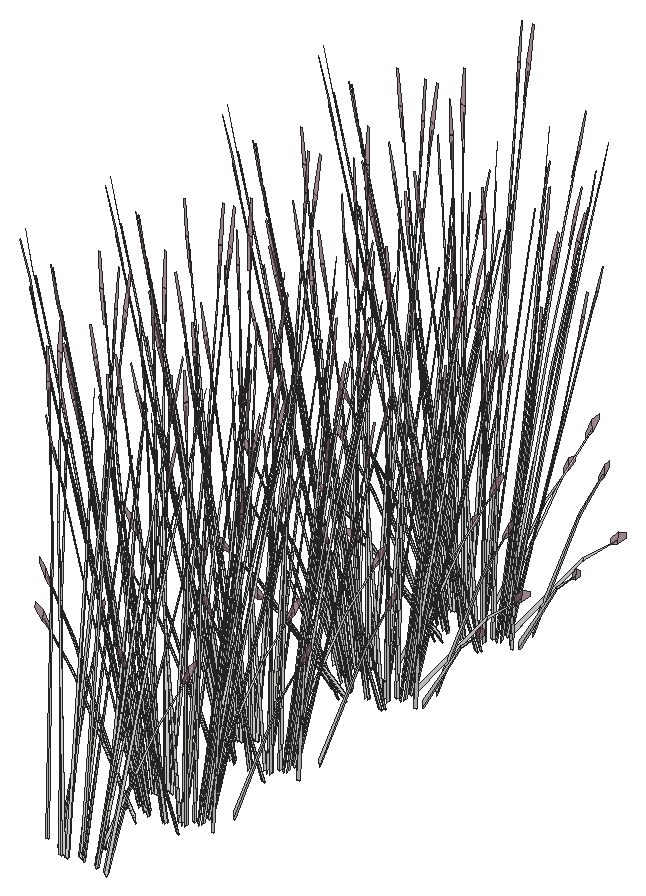
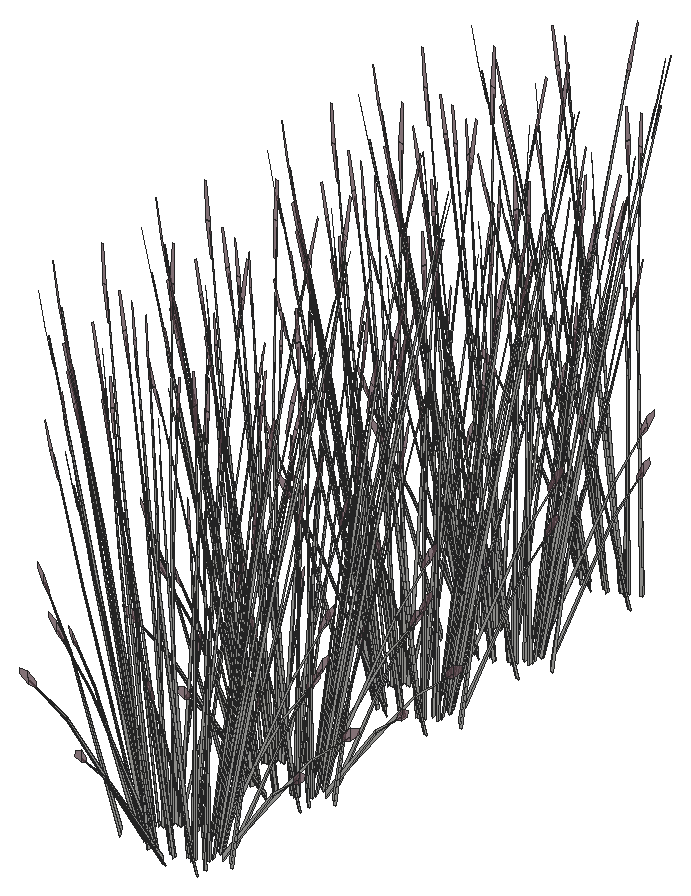
# SketchUp Ruby script. Lengths in inches.
U = 1.inch
M = Sketchup.active_model
def pt(a) = Geom::Point3d.new(a.map { |v| v * U })
def face(e, loops, mat)
  f = e.add_face(loops[0].map { |a| pt(a) })
  loops[1..].each { |l| e.add_face(l.map { |a| pt(a) }).erase! }
  f.material = f.back_material = mat if mat
  f
end
# faces: each face lists its corners as indices into pts; further lists are holes
def faces(e, pts, list, mat = nil) = list.each { |f| face(e, (f[0].is_a?(Array) ? f : [f]).map { |l| l.map { |i| pts[i] } }, mat) }
# xy, xz, yz: faces in a plane at the given z, y or x. An outline is a flat list of corners, or four numbers for a rectangle; further outlines are holes
def ring(l) = l.size == 4 ? [[l[0], l[1]], [l[2], l[1]], [l[2], l[3]], [l[0], l[3]]] : l.each_slice(2).to_a
def flat(e, list, mat, &to3) = list.each { |f| face(e, (f[0].is_a?(Array) ? f : [f]).map { |l| ring(l).map { |u, v| to3.(u, v) } }, mat) }
def xy(e, z, list, mat = nil) = flat(e, list, mat) { |x, y| [x, y, z] }
def xz(e, y, list, mat = nil) = flat(e, list, mat) { |x, z| [x, y, z] }
def yz(e, x, list, mat = nil) = flat(e, list, mat) { |y, z| [x, y, z] }
def lines(e, pts, list) = list.each { |a, b| e.add_line(pt(pts[a]), pt(pts[b])) }
# prism: a flat outline (further loops are holes) pulled along v
def prism(e, loops, v, mat = nil)
  f = face(e, loops, mat); d = Geom::Vector3d.new(v.map { |x| x * U })
  f.pushpull(f.normal.samedirection?(d) ? d.length : -d.length)
end
def box(e, o, s, mat = nil) = prism(e, [[o, [o[0] + s[0], o[1], o[2]], [o[0] + s[0], o[1] + s[1], o[2]], [o[0], o[1] + s[1], o[2]]]], [0, 0, s[2]], mat)
def at(x, y, z, deg = 0) = Geom::Transformation.translation(pt([x, y, z])) * Geom::Transformation.rotation(ORIGIN, Z_AXIS, deg.degrees)
def axes(o, x, y, z) = Geom::Transformation.new([*x, 0, *y, 0, *z, 0, *pt(o).to_a, 1])
def part(name) = M.definitions.add(name)
# library, detail: a bought-in or finely detailed component or shape, given as its bounding box
def library(name, o, s) = part(name).tap { |d| box(d.entities, o, s) }
def detail(e, o, s) = box(e.add_group.entities, o, s)
def put(e, d, t, mat = nil) = e.add_instance(d, t).tap { |i| i.material = mat if mat }
def group(e, t, mat = nil) = e.add_group.tap { |g| g.transformation = t; g.material = mat if mat }.entities
root = M.entities
M.materials.add("LightPink_Translucent").color = [144, 107, 117]
M.materials["LightPink_Translucent"].alpha = 0.75
c1 = part("blade")
p = [[2.15,0.21,22],[0,0.17,0],[0.09,0.45,0],[2.18,0.31,22],[2.29,0.31,22],[0.38,0.45,0],
  [2.48,0.24,33],[2.49,0.24,33],[2.48,0.22,33]]
faces(c1.entities,p,[[0,1,2,3],[4,5,2,3],[6,3,4,7],[8,0,3,6]])
c2 = part("seeds")
p = [[0.3,-0.1,1.38],[-0.01,-0.03,1.59],[-0.01,-0.03,0.03],[0.14,-0.07,-0.07],[0.29,-0.03,3],[0.15,0.01,3.11]]
faces(c2.entities,p,[[0,1,2,3],[1,0,4,5]],"LightPink_Translucent")
c3 = part("blade with seeds")
put(c3.entities,c1,at(0,0,0))
put(c3.entities,c2,axes([2.4,0.25,30.99],[1.5799,-0.05474,1.17369],[-0.12525,1.92788,0.29478],[-0.07173,-0.02425,1.56792]))
put(root,c3,axes([335.62,462.02,52.18],[-0.02542,0.29714,0.05682],[-0.38391,-0.00815,0.44729],[0.14706,0.03109,0.68204]))
put(root,c3,axes([335.65,461.93,52.18],[-0.3723,0.25748,0.42415],[-0.32109,-0.27343,0.34973],[0.17467,0.04749,0.87768]))
put(root,c3,axes([330.85,462.21,52.99],[0.44556,0.1043,-0.05733],[-0.13706,0.32103,-0.25992],[-0.07288,0.04874,0.85731]))
put(root,c3,axes([334.47,462.22,52.46],[-0.07798,-0.31474,0.31292],[0.44579,-0.08311,-0.40398],[0.11974,0.09019,0.77298]))
put(root,c3,axes([332.45,461.94,52.46],[0.34164,-0.20573,0.31292],[0.3234,0.23491,-0.40398],[-0.04921,0.11936,0.77298]))
put(root,c3,axes([334.04,462.66,52.16],[0.00149,-0.04731,1.56736],[0.4327,-0.20872,-0.1481],[0.1503,0.0745,0.27737]))
put(root,c3,axes([332.14,462.12,52.18],[-0.41493,-0.01821,0.05682],[0.01138,-0.27493,0.44729],[-0.04342,0.10531,0.68204]))
put(root,c3,axes([332.27,462.15,52.18],[-0.35954,-0.26661,0.42415],[0.38183,-0.22994,0.34973],[-0.06632,0.12508,0.87768]))
put(root,c3,axes([333.4,462.27,52.46],[0.15222,-0.30049,0.31292],[0.44409,0.08764,-0.40398],[0.04072,0.12098,0.77298]))
put(root,c3,axes([334.54,462.51,52.18],[-0.22948,0.24822,0.05682],[-0.32679,-0.14452,0.44729],[0.10565,0.07958,0.68204]))
put(root,c3,axes([334,463.35,52.99],[0.34892,-0.22417,-0.05733],[0.3197,0.24551,-0.25992],[0.02251,0.06957,0.85731]))
put(root,c3,axes([334.64,462.44,52.18],[-0.5022,0.08967,0.42415],[-0.08716,-0.35177,0.34973],[0.11811,0.10367,0.87768]))
put(root,c3,axes([333.27,462.55,52.18],[-0.37205,0.1328,0.05682],[-0.18211,-0.24217,0.44729],[0.03593,0.10675,0.68204]))
put(root,c3,axes([332.23,461.99,52.77],[0.55492,0.01936,-0.11927],[-0.01517,0.36657,-0.66198],[-0.03855,0.14118,1.00587]))
put(root,c3,axes([333.4,462.52,52.47],[-0.49753,-0.10215,0.47081],[0.17013,-0.33585,0.3882],[0.0299,0.13207,0.97422]))
put(root,c3,axes([331.05,462.96,52.16],[0.05728,-0.02359,1.56736],[0.47345,0.15692,-0.1481],[-0.01113,0.13066,0.27737]))
put(root,c3,axes([335.78,468.35,52.16],[-0.05128,0.02985,1.56736],[-0.5024,-0.1007,-0.1481],[-0.01819,-0.13025,0.27737]))
put(root,c3,axes([333.05,467.78,52.16],[-0.00942,0.04684,1.56736],[-0.46458,0.16998,-0.1481],[-0.13671,-0.08689,0.27737]))
put(root,c3,axes([332.94,468.61,52.5],[0.56246,-0.10044,0.47505],[0.09762,0.39398,0.3917],[-0.13228,-0.11611,0.983]))
put(root,c3,axes([334.22,468.68,52.18],[0.49753,0.10215,0.42415],[-0.17013,0.33585,0.34973],[-0.0299,-0.13207,0.87768]))
put(root,c3,axes([334.35,468.66,52.18],[0.37205,-0.1328,0.05682],[0.18211,0.24217,0.44729],[-0.03593,-0.10675,0.68204]))
put(root,c3,axes([333.07,468.7,52.18],[0.22948,-0.24822,0.05682],[0.32679,0.14452,0.44729],[-0.10565,-0.07958,0.68204]))
put(root,c3,axes([334.21,468.93,52.46],[-0.15222,0.30049,0.31292],[-0.44409,-0.08764,-0.40398],[-0.04072,-0.12098,0.77298]))
put(root,c3,axes([335.34,469.06,52.18],[0.35954,0.26661,0.42415],[-0.38183,0.22994,0.34973],[0.06632,-0.12508,0.87768]))
put(root,c3,axes([333.18,468.67,52.8],[-0.33698,0.3746,-0.12034],[-0.48801,-0.21581,-0.66795],[-0.16964,-0.10584,1.01494]))
put(root,c3,axes([335.48,469.08,52.18],[0.41493,0.01821,0.05682],[-0.01138,0.27493,0.44729],[0.04342,-0.10531,0.68204]))
put(root,c3,axes([335.17,469.27,52.46],[-0.34164,0.20573,0.31292],[-0.3234,-0.23491,-0.40398],[0.04921,-0.11936,0.77298]))
put(root,c3,axes([333.14,468.98,52.46],[0.07798,0.31474,0.31292],[-0.44579,0.08311,-0.40398],[-0.11974,-0.09019,0.77298]))
put(root,c3,axes([331.8,469.1875,52.5],[0.41698,-0.28837,0.47505],[0.35962,0.30624,0.3917],[-0.19563,-0.05319,0.983]))
put(root,c3,axes([337.14,469.84,52.16],[-0.06595,-0.00297,1.56736],[-0.27386,-0.31799,-0.1481],[0.10998,-0.10455,0.27737]))
put(root,c3,axes([331.99,469.18,52.18],[0.02542,-0.29714,0.05682],[0.38391,0.00815,0.44729],[-0.14706,-0.03109,0.68204]))
put(root,c3,axes([335.76,469.91,52.46],[-0.43951,0.05584,0.31292],[-0.11606,-0.31924,-0.40398],[0.12595,-0.08575,0.77298]))
put(root,c3,axes([336.16,469.85,52.18],[0.34663,0.16434,0.05682],[-0.20181,0.23402,0.44729],[0.11113,-0.07566,0.68204]))
put(root,c3,axes([336.0625,469.79,52.18],[0.12522,0.35963,0.42415],[-0.49122,0.06241,0.34973],[0.14477,-0.08458,0.87768]))
put(root,c3,axes([331.47,468.8,52.16],[0.03743,0.039,1.56736],[-0.18045,0.35054,-0.1481],[-0.18276,0.00254,0.27737]))
put(root,c3,axes([332.25,469.41,52.46],[0.28729,0.24465,0.31292],[-0.32804,0.23159,-0.40398],[-0.16667,-0.03524,0.77298]))
put(root,c3,axes([335.83,470.67,52.46],[-0.41962,-0.10901,0.31292],[0.12239,-0.31802,-0.40398],[0.16894,-0.02916,0.77298]))
put(root,c3,axes([331.4375,470.09,52.18],[0.14265,-0.35629,0.42415],[0.46898,0.12183,0.34973],[-0.18443,0.02141,0.87768]))
put(root,c3,axes([331.4,469.99,52.18],[-0.18545,-0.26643,0.05682],[0.33817,-0.13041,0.44729],[-0.14907,0.02573,0.68204]))
put(root,c3,axes([336.21,470.77,52.18],[0.18545,0.26643,0.05682],[-0.33817,0.13041,0.44729],[0.14907,-0.02573,0.68204]))
put(root,c3,axes([336.18,470.67,52.18],[-0.14265,0.35629,0.42415],[-0.46898,-0.12183,0.34973],[0.18443,-0.02141,0.87768]))
put(root,c3,axes([331.78,470.09,52.46],[0.41962,0.10901,0.31292],[-0.12239,0.31802,-0.40398],[-0.16894,0.02916,0.77298]))
put(root,c3,axes([337.02,471.83,52.16],[-0.04566,-0.03421,1.56736],[0.09987,-0.36669,-0.1481],[0.17984,-0.02343,0.27737]))
put(root,c3,axes([335.36,471.35,52.46],[-0.28729,-0.24465,0.31292],[0.32804,-0.23159,-0.40398],[0.16667,0.03524,0.77298]))
put(root,c3,axes([331.55,470.97,52.18],[-0.12522,-0.35963,0.42415],[0.49122,-0.06241,0.34973],[-0.14477,0.08458,0.87768]))
put(root,c3,axes([331.45,470.91,52.18],[-0.34663,-0.16434,0.05682],[0.20181,-0.23402,0.44729],[-0.11113,0.07566,0.68204]))
put(root,c3,axes([331.85,470.86,52.46],[0.43951,-0.05584,0.31292],[0.11606,0.31924,-0.40398],[-0.12595,0.08575,0.77298]))
put(root,c3,axes([330.16,470.71,52.16],[0.06444,0.01048,1.56736],[0.19934,0.34525,-0.1481],[-0.13191,0.09062,0.27737]))
put(root,c3,axes([335.62,471.58,52.18],[-0.02542,0.29714,0.05682],[-0.38391,-0.00815,0.44729],[0.14706,0.03109,0.68204]))
put(root,c3,axes([335.65,471.48,52.18],[-0.3723,0.25748,0.42415],[-0.32109,-0.27343,0.34973],[0.17467,0.04749,0.87768]))
put(root,c3,axes([330.85,471.76,52.99],[0.44556,0.1043,-0.05733],[-0.13706,0.32103,-0.25992],[-0.07288,0.04874,0.85731]))
put(root,c3,axes([334.47,471.78,52.46],[-0.07798,-0.31474,0.31292],[0.44579,-0.08311,-0.40398],[0.11974,0.09019,0.77298]))
put(root,c3,axes([332.45,471.49,52.46],[0.34164,-0.20573,0.31292],[0.3234,0.23491,-0.40398],[-0.04921,0.11936,0.77298]))
put(root,c3,axes([334.04,472.22,52.16],[0.00149,-0.04731,1.56736],[0.4327,-0.20872,-0.1481],[0.1503,0.0745,0.27737]))
put(root,c3,axes([332.14,471.68,52.18],[-0.41493,-0.01821,0.05682],[0.01138,-0.27493,0.44729],[-0.04342,0.10531,0.68204]))
put(root,c3,axes([332.27,471.7,52.18],[-0.35954,-0.26661,0.42415],[0.38183,-0.22994,0.34973],[-0.06632,0.12508,0.87768]))
put(root,c3,axes([333.4,471.83,52.46],[0.15222,-0.30049,0.31292],[0.44409,0.08764,-0.40398],[0.04072,0.12098,0.77298]))
put(root,c3,axes([335.78,476.15,52.16],[-0.05128,0.02985,1.56736],[-0.5024,-0.1007,-0.1481],[-0.01819,-0.13025,0.27737]))
put(root,c3,axes([334.54,472.06,52.18],[-0.22948,0.24822,0.05682],[-0.32679,-0.14452,0.44729],[0.10565,0.07958,0.68204]))
put(root,c3,axes([334,472.9,52.99],[0.34892,-0.22417,-0.05733],[0.3197,0.24551,-0.25992],[0.02251,0.06957,0.85731]))
put(root,c3,axes([334.64,472,52.18],[-0.5022,0.08967,0.42415],[-0.08716,-0.35177,0.34973],[0.11811,0.10367,0.87768]))
put(root,c3,axes([333.05,475.58,52.16],[-0.00942,0.04684,1.56736],[-0.46458,0.16998,-0.1481],[-0.13671,-0.08689,0.27737]))
put(root,c3,axes([333.27,472.1,52.18],[-0.37205,0.1328,0.05682],[-0.18211,-0.24217,0.44729],[0.03593,0.10675,0.68204]))
put(root,c3,axes([332.23,471.55,52.77],[0.55492,0.01936,-0.11927],[-0.01517,0.36657,-0.66198],[-0.03855,0.14118,1.00587]))
put(root,c3,axes([332.94,476.41,52.5],[0.56246,-0.10044,0.47505],[0.09762,0.39398,0.3917],[-0.13228,-0.11611,0.983]))
put(root,c3,axes([333.4,472.08,52.47],[-0.49753,-0.10215,0.47081],[0.17013,-0.33585,0.3882],[0.0299,0.13207,0.97422]))
put(root,c3,axes([334.22,476.48,52.18],[0.49753,0.10215,0.42415],[-0.17013,0.33585,0.34973],[-0.0299,-0.13207,0.87768]))
put(root,c3,axes([334.35,476.46,52.18],[0.37205,-0.1328,0.05682],[0.18211,0.24217,0.44729],[-0.03593,-0.10675,0.68204]))
put(root,c3,axes([333.07,476.49,52.18],[0.22948,-0.24822,0.05682],[0.32679,0.14452,0.44729],[-0.10565,-0.07958,0.68204]))
put(root,c3,axes([331.05,472.52,52.16],[0.05728,-0.02359,1.56736],[0.47345,0.15692,-0.1481],[-0.01113,0.13066,0.27737]))
put(root,c3,axes([334.21,476.73,52.46],[-0.15222,0.30049,0.31292],[-0.44409,-0.08764,-0.40398],[-0.04072,-0.12098,0.77298]))
put(root,c3,axes([335.34,476.85,52.18],[0.35954,0.26661,0.42415],[-0.38183,0.22994,0.34973],[0.06632,-0.12508,0.87768]))
put(root,c3,axes([333.18,476.47,52.8],[-0.33698,0.3746,-0.12034],[-0.48801,-0.21581,-0.66795],[-0.16964,-0.10584,1.01494]))
put(root,c3,axes([335.48,476.88,52.18],[0.41493,0.01821,0.05682],[-0.01138,0.27493,0.44729],[0.04342,-0.10531,0.68204]))
put(root,c3,axes([335.17,477.07,52.46],[-0.34164,0.20573,0.31292],[-0.3234,-0.23491,-0.40398],[0.04921,-0.11936,0.77298]))
put(root,c3,axes([333.14,476.78,52.46],[0.07798,0.31474,0.31292],[-0.44579,0.08311,-0.40398],[-0.11974,-0.09019,0.77298]))
put(root,c3,axes([331.8,476.98,52.5],[0.41698,-0.28837,0.47505],[0.35962,0.30624,0.3917],[-0.19563,-0.05319,0.983]))
put(root,c3,axes([337.14,477.64,52.16],[-0.06595,-0.00297,1.56736],[-0.27386,-0.31799,-0.1481],[0.10998,-0.10455,0.27737]))
put(root,c3,axes([331.99,476.98,52.18],[0.02542,-0.29714,0.05682],[0.38391,0.00815,0.44729],[-0.14706,-0.03109,0.68204]))
put(root,c3,axes([335.76,477.7,52.46],[-0.43951,0.05584,0.31292],[-0.11606,-0.31924,-0.40398],[0.12595,-0.08575,0.77298]))
put(root,c3,axes([336.16,477.65,52.18],[0.34663,0.16434,0.05682],[-0.20181,0.23402,0.44729],[0.11113,-0.07566,0.68204]))
put(root,c3,axes([336.0625,477.58,52.18],[0.12522,0.35963,0.42415],[-0.49122,0.06241,0.34973],[0.14477,-0.08458,0.87768]))
put(root,c3,axes([331.47,476.59,52.16],[0.03743,0.039,1.56736],[-0.18045,0.35054,-0.1481],[-0.18276,0.00254,0.27737]))
put(root,c3,axes([332.25,477.2,52.46],[0.28729,0.24465,0.31292],[-0.32804,0.23159,-0.40398],[-0.16667,-0.03524,0.77298]))
put(root,c3,axes([335.83,478.47,52.46],[-0.41962,-0.10901,0.31292],[0.12239,-0.31802,-0.40398],[0.16894,-0.02916,0.77298]))
put(root,c3,axes([331.4375,477.88,52.18],[0.14265,-0.35629,0.42415],[0.46898,0.12183,0.34973],[-0.18443,0.02141,0.87768]))
put(root,c3,axes([331.4,477.79,52.18],[-0.18545,-0.26643,0.05682],[0.33817,-0.13041,0.44729],[-0.14907,0.02573,0.68204]))
put(root,c3,axes([336.21,478.5625,52.18],[0.18545,0.26643,0.05682],[-0.33817,0.13041,0.44729],[0.14907,-0.02573,0.68204]))
put(root,c3,axes([336.18,478.47,52.18],[-0.14265,0.35629,0.42415],[-0.46898,-0.12183,0.34973],[0.18443,-0.02141,0.87768]))
put(root,c3,axes([331.78,477.89,52.46],[0.41962,0.10901,0.31292],[-0.12239,0.31802,-0.40398],[-0.16894,0.02916,0.77298]))
put(root,c3,axes([337.02,479.625,52.16],[-0.04566,-0.03421,1.56736],[0.09987,-0.36669,-0.1481],[0.17984,-0.02343,0.27737]))
put(root,c3,axes([335.36,479.15,52.46],[-0.28729,-0.24465,0.31292],[0.32804,-0.23159,-0.40398],[0.16667,0.03524,0.77298]))
put(root,c3,axes([331.55,478.77,52.18],[-0.12522,-0.35963,0.42415],[0.49122,-0.06241,0.34973],[-0.14477,0.08458,0.87768]))
put(root,c3,axes([331.45,478.7,52.18],[-0.34663,-0.16434,0.05682],[0.20181,-0.23402,0.44729],[-0.11113,0.07566,0.68204]))
put(root,c3,axes([331.85,478.65,52.46],[0.43951,-0.05584,0.31292],[0.11606,0.31924,-0.40398],[-0.12595,0.08575,0.77298]))
put(root,c3,axes([330.16,478.51,52.16],[0.06444,0.01048,1.56736],[0.19934,0.34525,-0.1481],[-0.13191,0.09062,0.27737]))
put(root,c3,axes([335.62,479.375,52.18],[-0.02542,0.29714,0.05682],[-0.38391,-0.00815,0.44729],[0.14706,0.03109,0.68204]))
put(root,c3,axes([335.65,479.28,52.18],[-0.3723,0.25748,0.42415],[-0.32109,-0.27343,0.34973],[0.17467,0.04749,0.87768]))
put(root,c3,axes([330.85,479.56,52.99],[0.44556,0.1043,-0.05733],[-0.13706,0.32103,-0.25992],[-0.07288,0.04874,0.85731]))
put(root,c3,axes([334.47,479.58,52.46],[-0.07798,-0.31474,0.31292],[0.44579,-0.08311,-0.40398],[0.11974,0.09019,0.77298]))
put(root,c3,axes([332.45,479.29,52.46],[0.34164,-0.20573,0.31292],[0.3234,0.23491,-0.40398],[-0.04921,0.11936,0.77298]))
put(root,c3,axes([334.04,480.02,52.16],[0.00149,-0.04731,1.56736],[0.4327,-0.20872,-0.1481],[0.1503,0.0745,0.27737]))
put(root,c3,axes([332.14,479.47,52.18],[-0.41493,-0.01821,0.05682],[0.01138,-0.27493,0.44729],[-0.04342,0.10531,0.68204]))
put(root,c3,axes([332.27,479.5,52.18],[-0.35954,-0.26661,0.42415],[0.38183,-0.22994,0.34973],[-0.06632,0.12508,0.87768]))
put(root,c3,axes([333.4,479.625,52.46],[0.15222,-0.30049,0.31292],[0.44409,0.08764,-0.40398],[0.04072,0.12098,0.77298]))
put(root,c3,axes([334.54,479.86,52.18],[-0.22948,0.24822,0.05682],[-0.32679,-0.14452,0.44729],[0.10565,0.07958,0.68204]))
put(root,c3,axes([334,480.7,52.99],[0.34892,-0.22417,-0.05733],[0.3197,0.24551,-0.25992],[0.02251,0.06957,0.85731]))
put(root,c3,axes([334.64,479.79,52.18],[-0.5022,0.08967,0.42415],[-0.08716,-0.35177,0.34973],[0.11811,0.10367,0.87768]))
put(root,c3,axes([333.27,479.9,52.18],[-0.37205,0.1328,0.05682],[-0.18211,-0.24217,0.44729],[0.03593,0.10675,0.68204]))
put(root,c3,axes([332.23,479.34,52.77],[0.55492,0.01936,-0.11927],[-0.01517,0.36657,-0.66198],[-0.03855,0.14118,1.00587]))
put(root,c3,axes([333.4,479.875,52.47],[-0.49753,-0.10215,0.47081],[0.17013,-0.33585,0.3882],[0.0299,0.13207,0.97422]))
put(root,c3,axes([331.05,480.3125,52.16],[0.05728,-0.02359,1.56736],[0.47345,0.15692,-0.1481],[-0.01113,0.13066,0.27737]))
put(root,c3,axes([333.57,486.46,52.17],[-0.07723,-0.05479,1.54581],[-0.51538,0.03473,-0.24447],[-0.08225,-0.13104,0.12397]))
put(root,c3,axes([335.89,487.13,52.17],[-0.00487,-0.07777,1.54581],[-0.41166,-0.22476,-0.24447],[0.06364,-0.13625,0.12397]))
put(root,c3,axes([335.78,486.85,52.16],[-0.05128,0.02985,1.56736],[-0.5024,-0.1007,-0.1481],[-0.01819,-0.13025,0.27737]))
put(root,c3,axes([333.05,486.28,52.16],[-0.00942,0.04684,1.56736],[-0.46458,0.16998,-0.1481],[-0.13671,-0.08689,0.27737]))
put(root,c3,axes([332.94,487.11,52.5],[0.56246,-0.10044,0.47505],[0.09762,0.39398,0.3917],[-0.13228,-0.11611,0.983]))
put(root,c3,axes([334.22,487.18,52.18],[0.49753,0.10215,0.42415],[-0.17013,0.33585,0.34973],[-0.0299,-0.13207,0.87768]))
put(root,c3,axes([334.35,487.16,52.18],[0.37205,-0.1328,0.05682],[0.18211,0.24217,0.44729],[-0.03593,-0.10675,0.68204]))
put(root,c3,axes([333.07,487.19,52.18],[0.22948,-0.24822,0.05682],[0.32679,0.14452,0.44729],[-0.10565,-0.07958,0.68204]))
put(root,c3,axes([334.21,487.43,52.46],[-0.15222,0.30049,0.31292],[-0.44409,-0.08764,-0.40398],[-0.04072,-0.12098,0.77298]))
put(root,c3,axes([335.34,487.55,52.18],[0.35954,0.26661,0.42415],[-0.38183,0.22994,0.34973],[0.06632,-0.12508,0.87768]))
put(root,c3,axes([333.18,487.17,52.8],[-0.33698,0.3746,-0.12034],[-0.48801,-0.21581,-0.66795],[-0.16964,-0.10584,1.01494]))
put(root,c3,axes([335.48,487.58,52.18],[0.41493,0.01821,0.05682],[-0.01138,0.27493,0.44729],[0.04342,-0.10531,0.68204]))
put(root,c3,axes([335.17,487.77,52.46],[-0.34164,0.20573,0.31292],[-0.3234,-0.23491,-0.40398],[0.04921,-0.11936,0.77298]))
put(root,c3,axes([331.88,487.06,52.17],[-0.10864,-0.00276,1.54581],[-0.34587,0.27582,-0.24447],[-0.18454,-0.05636,0.12397]))
put(root,c3,axes([333.14,487.48,52.46],[0.07798,0.31474,0.31292],[-0.44579,0.08311,-0.40398],[-0.11974,-0.09019,0.77298]))
put(root,c3,axes([331.8,487.68,52.5],[0.41698,-0.28837,0.47505],[0.35962,0.30624,0.3917],[-0.19563,-0.05319,0.983]))
put(root,c3,axes([337.14,488.34,52.16],[-0.06595,-0.00297,1.56736],[-0.27386,-0.31799,-0.1481],[0.10998,-0.10455,0.27737]))
put(root,c3,axes([331.99,487.68,52.18],[0.02542,-0.29714,0.05682],[0.38391,0.00815,0.44729],[-0.14706,-0.03109,0.68204]))
put(root,c3,axes([335.76,488.4,52.46],[-0.43951,0.05584,0.31292],[-0.11606,-0.31924,-0.40398],[0.12595,-0.08575,0.77298]))
put(root,c3,axes([336.16,488.35,52.18],[0.34663,0.16434,0.05682],[-0.20181,0.23402,0.44729],[0.11113,-0.07566,0.68204]))
put(root,c3,axes([336.0625,488.28,52.18],[0.12522,0.35963,0.42415],[-0.49122,0.06241,0.34973],[0.14477,-0.08458,0.87768]))
put(root,c3,axes([337.39,488.72,52.17],[0.07006,-0.05952,1.54581],[-0.08968,-0.3651,-0.24447],[0.1758,-0.06922,0.12397]))
put(root,c3,axes([331.47,487.29,52.16],[0.03743,0.039,1.56736],[-0.18045,0.35054,-0.1481],[-0.18276,0.00254,0.27737]))
put(root,c3,axes([332.25,487.9,52.46],[0.28729,0.24465,0.31292],[-0.32804,0.23159,-0.40398],[-0.16667,-0.03524,0.77298]))
put(root,c3,axes([335.83,489.17,52.46],[-0.41962,-0.10901,0.31292],[0.12239,-0.31802,-0.40398],[0.16894,-0.02916,0.77298]))
put(root,c3,axes([331.4375,488.58,52.18],[0.14265,-0.35629,0.42415],[0.46898,0.12183,0.34973],[-0.18443,0.02141,0.87768]))
put(root,c3,axes([331.4,488.49,52.18],[-0.18545,-0.26643,0.05682],[0.33817,-0.13041,0.44729],[-0.14907,0.02573,0.68204]))
put(root,c3,axes([336.21,489.26,52.18],[0.18545,0.26643,0.05682],[-0.33817,0.13041,0.44729],[0.14907,-0.02573,0.68204]))
put(root,c3,axes([336.18,489.17,52.18],[-0.14265,0.35629,0.42415],[-0.46898,-0.12183,0.34973],[0.18443,-0.02141,0.87768]))
put(root,c3,axes([331.78,488.59,52.46],[0.41962,0.10901,0.31292],[-0.12239,0.31802,-0.40398],[-0.16894,0.02916,0.77298]))
put(root,c3,axes([337.02,490.32,52.16],[-0.04566,-0.03421,1.56736],[0.09987,-0.36669,-0.1481],[0.17984,-0.02343,0.27737]))
put(root,c3,axes([331.08,488.84,52.17],[-0.08245,0.05073,1.54581],[0.00701,0.37067,-0.24447],[-0.18899,0.0482,0.12397]))
put(root,c3,axes([335.36,489.85,52.46],[-0.28729,-0.24465,0.31292],[0.32804,-0.23159,-0.40398],[0.16667,0.03524,0.77298]))
put(root,c3,axes([335.88,489.77,52.17],[0.10831,-0.00661,1.54581],[0.29709,-0.30358,-0.24447],[0.19266,0.04007,0.12397]))
put(root,c3,axes([331.55,489.47,52.18],[-0.12522,-0.35963,0.42415],[0.49122,-0.06241,0.34973],[-0.14477,0.08458,0.87768]))
put(root,c3,axes([331.45,489.4,52.18],[-0.34663,-0.16434,0.05682],[0.20181,-0.23402,0.44729],[-0.11113,0.07566,0.68204]))
put(root,c3,axes([331.85,489.35,52.46],[0.43951,-0.05584,0.31292],[0.11606,0.31924,-0.40398],[-0.12595,0.08575,0.77298]))
put(root,c3,axes([330.16,489.21,52.16],[0.06444,0.01048,1.56736],[0.19934,0.34525,-0.1481],[-0.13191,0.09062,0.27737]))
put(root,c3,axes([335.62,490.07,52.18],[-0.02542,0.29714,0.05682],[-0.38391,-0.00815,0.44729],[0.14706,0.03109,0.68204]))
put(root,c3,axes([335.65,489.98,52.18],[-0.3723,0.25748,0.42415],[-0.32109,-0.27343,0.34973],[0.17467,0.04749,0.87768]))
put(root,c3,axes([330.85,490.26,52.99],[0.44556,0.1043,-0.05733],[-0.13706,0.32103,-0.25992],[-0.07288,0.04874,0.85731]))
put(root,c3,axes([334.47,490.28,52.46],[-0.07798,-0.31474,0.31292],[0.44579,-0.08311,-0.40398],[0.11974,0.09019,0.77298]))
put(root,c3,axes([332.45,489.99,52.46],[0.34164,-0.20573,0.31292],[0.3234,0.23491,-0.40398],[-0.04921,0.11936,0.77298]))
put(root,c3,axes([334.04,490.72,52.16],[0.00149,-0.04731,1.56736],[0.4327,-0.20872,-0.1481],[0.1503,0.0745,0.27737]))
put(root,c3,axes([332.14,490.17,52.18],[-0.41493,-0.01821,0.05682],[0.01138,-0.27493,0.44729],[-0.04342,0.10531,0.68204]))
put(root,c3,axes([332.27,490.2,52.18],[-0.35954,-0.26661,0.42415],[0.38183,-0.22994,0.34973],[-0.06632,0.12508,0.87768]))
put(root,c3,axes([333.4,490.33,52.46],[0.15222,-0.30049,0.31292],[0.44409,0.08764,-0.40398],[0.04072,0.12098,0.77298]))
put(root,c3,axes([334.54,490.5625,52.18],[-0.22948,0.24822,0.05682],[-0.32679,-0.14452,0.44729],[0.10565,0.07958,0.68204]))
put(root,c3,axes([334,491.4,52.99],[0.34892,-0.22417,-0.05733],[0.3197,0.24551,-0.25992],[0.02251,0.06957,0.85731]))
put(root,c3,axes([334.64,490.49,52.18],[-0.5022,0.08967,0.42415],[-0.08716,-0.35177,0.34973],[0.11811,0.10367,0.87768]))
put(root,c3,axes([333.27,490.6,52.18],[-0.37205,0.1328,0.05682],[-0.18211,-0.24217,0.44729],[0.03593,0.10675,0.68204]))
put(root,c3,axes([331.09,490.22,52.17],[-0.01255,0.07733,1.54581],[0.35618,0.269,-0.24447],[-0.09325,0.12721,0.12397]))
put(root,c3,axes([332.23,490.04,52.77],[0.55492,0.01936,-0.11927],[-0.01517,0.36657,-0.66198],[-0.03855,0.14118,1.00587]))
put(root,c3,axes([333.4,490.57,52.47],[-0.49753,-0.10215,0.47081],[0.17013,-0.33585,0.3882],[0.0299,0.13207,0.97422]))
put(root,c3,axes([333.57,495.23,52.17],[-0.07723,-0.05479,1.54581],[-0.51538,0.03473,-0.24447],[-0.08225,-0.13104,0.12397]))
put(root,c3,axes([335.89,495.9,52.17],[-0.00487,-0.07777,1.54581],[-0.41166,-0.22476,-0.24447],[0.06364,-0.13625,0.12397]))
put(root,c3,axes([335.78,495.625,52.16],[-0.05128,0.02985,1.56736],[-0.5024,-0.1007,-0.1481],[-0.01819,-0.13025,0.27737]))
put(root,c3,axes([331.05,491.01,52.16],[0.05728,-0.02359,1.56736],[0.47345,0.15692,-0.1481],[-0.01113,0.13066,0.27737]))
put(root,c3,axes([333.05,495.05,52.16],[-0.00942,0.04684,1.56736],[-0.46458,0.16998,-0.1481],[-0.13671,-0.08689,0.27737]))
put(root,c3,axes([332.94,495.88,52.5],[0.56246,-0.10044,0.47505],[0.09762,0.39398,0.3917],[-0.13228,-0.11611,0.983]))
put(root,c3,axes([334.22,495.96,52.18],[0.49753,0.10215,0.42415],[-0.17013,0.33585,0.34973],[-0.0299,-0.13207,0.87768]))
put(root,c3,axes([333.14,491.18,52.17],[0.064,0.06292,1.54581],[0.51651,0.02472,-0.24447],[0.05194,0.13877,0.12397]))
put(root,c3,axes([334.35,495.93,52.18],[0.37205,-0.1328,0.05682],[0.18211,0.24217,0.44729],[-0.03593,-0.10675,0.68204]))
put(root,c3,axes([333.07,495.97,52.18],[0.22948,-0.24822,0.05682],[0.32679,0.14452,0.44729],[-0.10565,-0.07958,0.68204]))
put(root,c3,axes([334.21,496.21,52.46],[-0.15222,0.30049,0.31292],[-0.44409,-0.08764,-0.40398],[-0.04072,-0.12098,0.77298]))
put(root,c3,axes([335.34,496.33,52.18],[0.35954,0.26661,0.42415],[-0.38183,0.22994,0.34973],[0.06632,-0.12508,0.87768]))
put(root,c3,axes([333.18,495.94,52.8],[-0.33698,0.3746,-0.12034],[-0.48801,-0.21581,-0.66795],[-0.16964,-0.10584,1.01494]))
put(root,c3,axes([335.48,496.36,52.18],[0.41493,0.01821,0.05682],[-0.01138,0.27493,0.44729],[0.04342,-0.10531,0.68204]))
put(root,c3,axes([335.17,496.54,52.46],[-0.34164,0.20573,0.31292],[-0.3234,-0.23491,-0.40398],[0.04921,-0.11936,0.77298]))
put(root,c3,axes([331.88,495.84,52.17],[-0.10864,-0.00276,1.54581],[-0.34587,0.27582,-0.24447],[-0.18454,-0.05636,0.12397]))
put(root,c3,axes([333.14,496.26,52.46],[0.07798,0.31474,0.31292],[-0.44579,0.08311,-0.40398],[-0.11974,-0.09019,0.77298]))
put(root,c3,axes([331.8,496.46,52.5],[0.41698,-0.28837,0.47505],[0.35962,0.30624,0.3917],[-0.19563,-0.05319,0.983]))
put(root,c3,axes([337.14,497.12,52.16],[-0.06595,-0.00297,1.56736],[-0.27386,-0.31799,-0.1481],[0.10998,-0.10455,0.27737]))
put(root,c3,axes([331.99,496.46,52.18],[0.02542,-0.29714,0.05682],[0.38391,0.00815,0.44729],[-0.14706,-0.03109,0.68204]))
put(root,c3,axes([335.76,497.18,52.46],[-0.43951,0.05584,0.31292],[-0.11606,-0.31924,-0.40398],[0.12595,-0.08575,0.77298]))
put(root,c3,axes([336.16,497.13,52.18],[0.34663,0.16434,0.05682],[-0.20181,0.23402,0.44729],[0.11113,-0.07566,0.68204]))
put(root,c3,axes([336.0625,497.06,52.18],[0.12522,0.35963,0.42415],[-0.49122,0.06241,0.34973],[0.14477,-0.08458,0.87768]))
put(root,c3,axes([337.39,497.5,52.17],[0.07006,-0.05952,1.54581],[-0.08968,-0.3651,-0.24447],[0.1758,-0.06922,0.12397]))
put(root,c3,axes([331.47,496.07,52.16],[0.03743,0.039,1.56736],[-0.18045,0.35054,-0.1481],[-0.18276,0.00254,0.27737]))
put(root,c3,axes([332.25,496.68,52.46],[0.28729,0.24465,0.31292],[-0.32804,0.23159,-0.40398],[-0.16667,-0.03524,0.77298]))
put(root,c3,axes([335.83,497.94,52.46],[-0.41962,-0.10901,0.31292],[0.12239,-0.31802,-0.40398],[0.16894,-0.02916,0.77298]))
put(root,c3,axes([331.4375,497.36,52.18],[0.14265,-0.35629,0.42415],[0.46898,0.12183,0.34973],[-0.18443,0.02141,0.87768]))
put(root,c3,axes([331.4,497.27,52.18],[-0.18545,-0.26643,0.05682],[0.33817,-0.13041,0.44729],[-0.14907,0.02573,0.68204]))
put(root,c3,axes([336.21,498.04,52.18],[0.18545,0.26643,0.05682],[-0.33817,0.13041,0.44729],[0.14907,-0.02573,0.68204]))
put(root,c3,axes([336.18,497.95,52.18],[-0.14265,0.35629,0.42415],[-0.46898,-0.12183,0.34973],[0.18443,-0.02141,0.87768]))
put(root,c3,axes([331.78,497.37,52.46],[0.41962,0.10901,0.31292],[-0.12239,0.31802,-0.40398],[-0.16894,0.02916,0.77298]))
put(root,c3,axes([337.02,499.1,52.16],[-0.04566,-0.03421,1.56736],[0.09987,-0.36669,-0.1481],[0.17984,-0.02343,0.27737]))
put(root,c3,axes([331.08,497.61,52.17],[-0.08245,0.05073,1.54581],[0.00701,0.37067,-0.24447],[-0.18899,0.0482,0.12397]))
put(root,c3,axes([335.36,498.63,52.46],[-0.28729,-0.24465,0.31292],[0.32804,-0.23159,-0.40398],[0.16667,0.03524,0.77298]))
put(root,c3,axes([335.88,498.55,52.17],[0.10831,-0.00661,1.54581],[0.29709,-0.30358,-0.24447],[0.19266,0.04007,0.12397]))
put(root,c3,axes([331.55,498.25,52.18],[-0.12522,-0.35963,0.42415],[0.49122,-0.06241,0.34973],[-0.14477,0.08458,0.87768]))
put(root,c3,axes([331.45,498.18,52.18],[-0.34663,-0.16434,0.05682],[0.20181,-0.23402,0.44729],[-0.11113,0.07566,0.68204]))
put(root,c3,axes([331.85,498.13,52.46],[0.43951,-0.05584,0.31292],[0.11606,0.31924,-0.40398],[-0.12595,0.08575,0.77298]))
put(root,c3,axes([330.16,497.99,52.16],[0.06444,0.01048,1.56736],[0.19934,0.34525,-0.1481],[-0.13191,0.09062,0.27737]))
put(root,c3,axes([335.62,498.85,52.18],[-0.02542,0.29714,0.05682],[-0.38391,-0.00815,0.44729],[0.14706,0.03109,0.68204]))
put(root,c3,axes([335.65,498.76,52.18],[-0.3723,0.25748,0.42415],[-0.32109,-0.27343,0.34973],[0.17467,0.04749,0.87768]))
put(root,c3,axes([330.85,499.04,52.99],[0.44556,0.1043,-0.05733],[-0.13706,0.32103,-0.25992],[-0.07288,0.04874,0.85731]))
put(root,c3,axes([334.47,499.05,52.46],[-0.07798,-0.31474,0.31292],[0.44579,-0.08311,-0.40398],[0.11974,0.09019,0.77298]))
put(root,c3,axes([332.45,498.77,52.46],[0.34164,-0.20573,0.31292],[0.3234,0.23491,-0.40398],[-0.04921,0.11936,0.77298]))
put(root,c3,axes([334.04,499.49,52.16],[0.00149,-0.04731,1.56736],[0.4327,-0.20872,-0.1481],[0.1503,0.0745,0.27737]))
put(root,c3,axes([332.14,498.95,52.18],[-0.41493,-0.01821,0.05682],[0.01138,-0.27493,0.44729],[-0.04342,0.10531,0.68204]))
put(root,c3,axes([332.27,498.98,52.18],[-0.35954,-0.26661,0.42415],[0.38183,-0.22994,0.34973],[-0.06632,0.12508,0.87768]))
put(root,c3,axes([333.4,499.1,52.46],[0.15222,-0.30049,0.31292],[0.44409,0.08764,-0.40398],[0.04072,0.12098,0.77298]))
put(root,c3,axes([334.54,499.34,52.18],[-0.22948,0.24822,0.05682],[-0.32679,-0.14452,0.44729],[0.10565,0.07958,0.68204]))
put(root,c3,axes([334,500.18,52.99],[0.34892,-0.22417,-0.05733],[0.3197,0.24551,-0.25992],[0.02251,0.06957,0.85731]))
put(root,c3,axes([334.64,499.27,52.18],[-0.5022,0.08967,0.42415],[-0.08716,-0.35177,0.34973],[0.11811,0.10367,0.87768]))
put(root,c3,axes([333.27,499.375,52.18],[-0.37205,0.1328,0.05682],[-0.18211,-0.24217,0.44729],[0.03593,0.10675,0.68204]))
put(root,c3,axes([331.09,499,52.17],[-0.01255,0.07733,1.54581],[0.35618,0.269,-0.24447],[-0.09325,0.12721,0.12397]))
put(root,c3,axes([332.23,498.82,52.77],[0.55492,0.01936,-0.11927],[-0.01517,0.36657,-0.66198],[-0.03855,0.14118,1.00587]))
put(root,c3,axes([333.4,499.35,52.47],[-0.49753,-0.10215,0.47081],[0.17013,-0.33585,0.3882],[0.0299,0.13207,0.97422]))
put(root,c3,axes([331.05,499.79,52.16],[0.05728,-0.02359,1.56736],[0.47345,0.15692,-0.1481],[-0.01113,0.13066,0.27737]))
put(root,c3,axes([333.14,499.95,52.17],[0.064,0.06292,1.54581],[0.51651,0.02472,-0.24447],[0.05194,0.13877,0.12397]))
